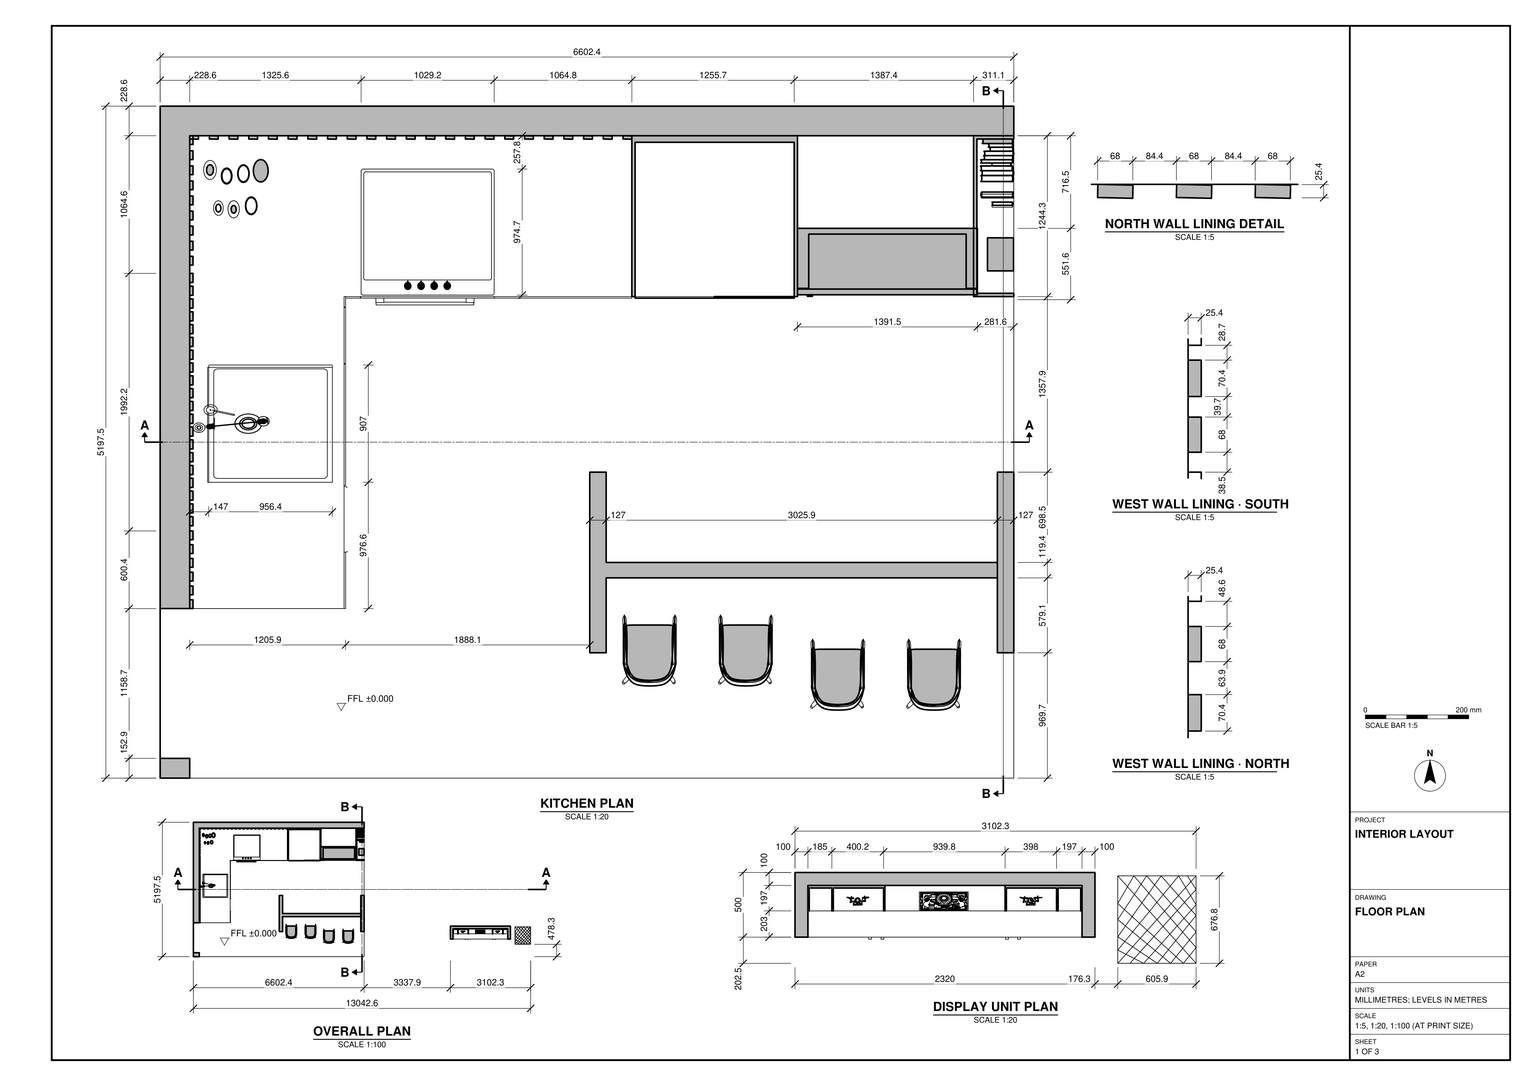
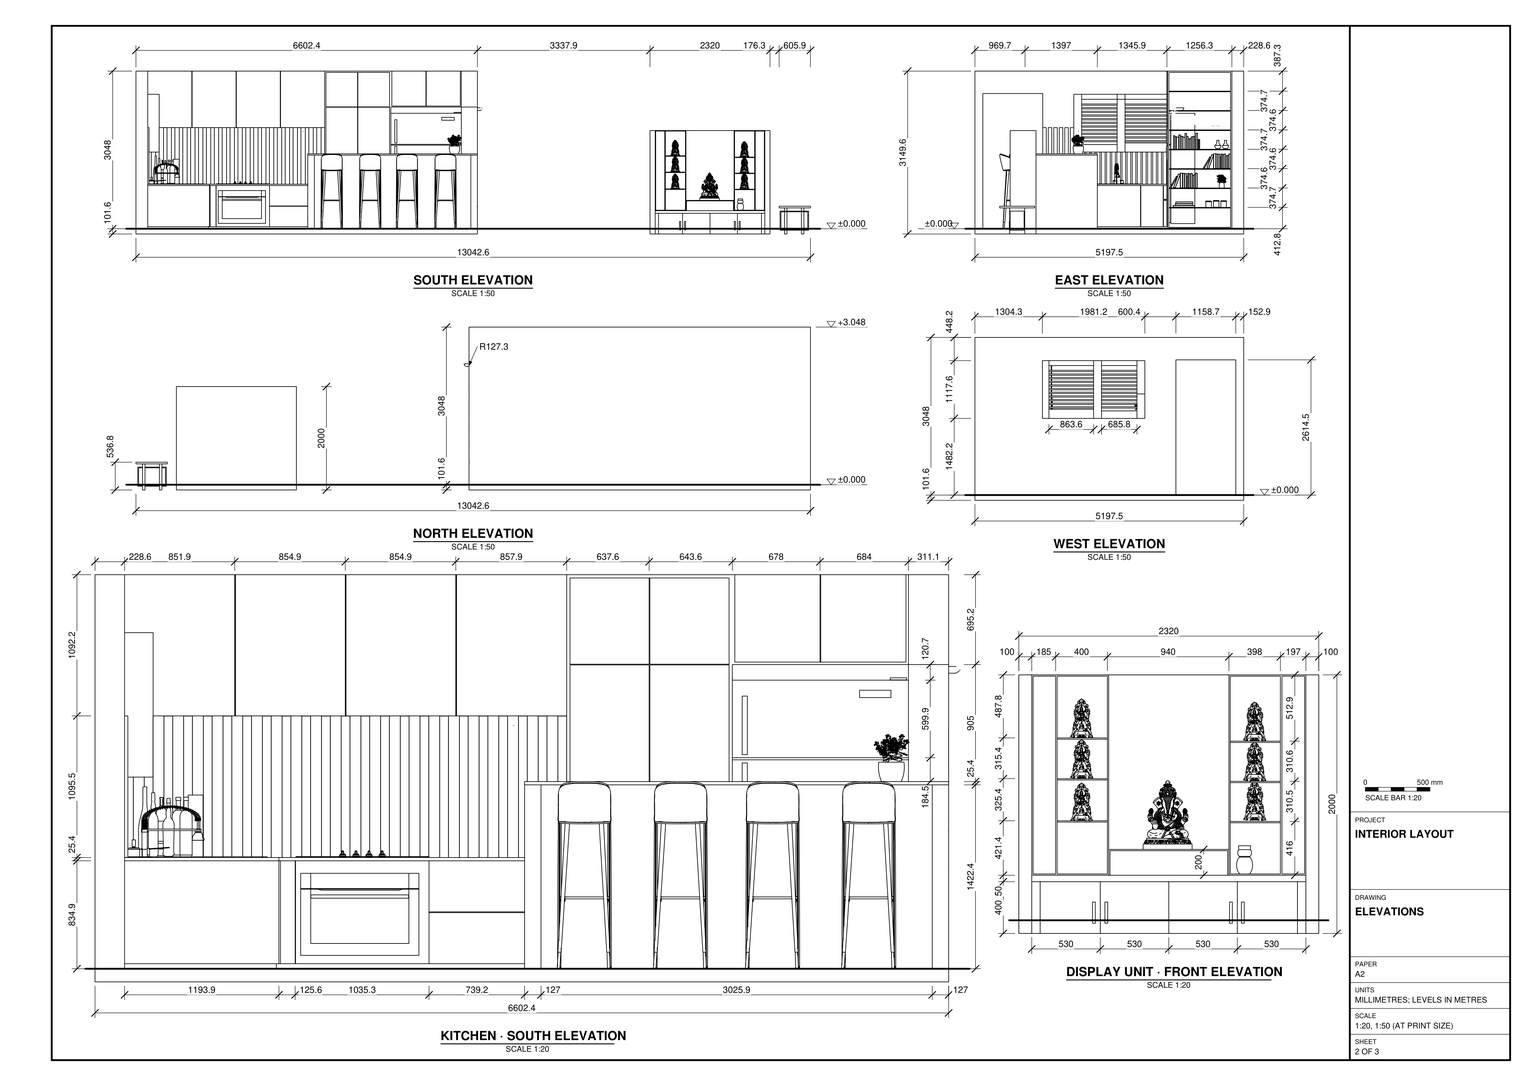
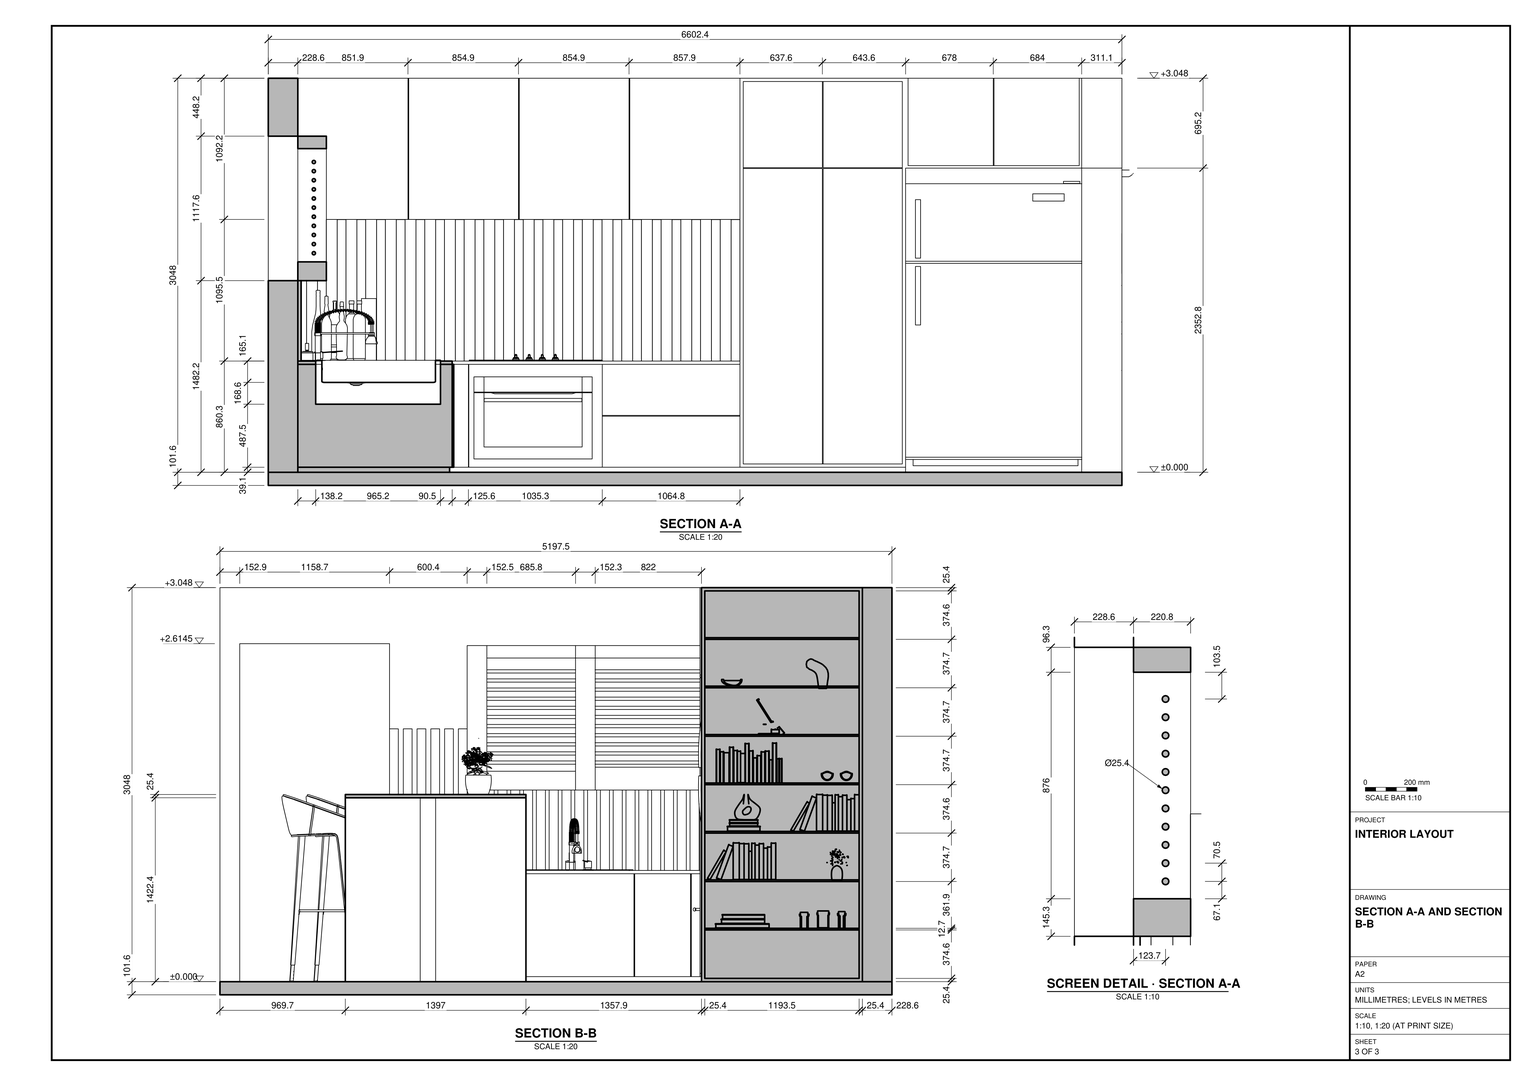
Build the interior in SketchUp from task_files/diagram_01.pdf. Work in millimetres and use the finished kitchen floor at ±0.000 (0 mm) as the level reference. The complete layout, including the display unit and the small table beyond it, measures 13042.6 mm along X, 5197.5 mm along Y and 3149.6 mm along Z.

Model the kitchen floor slab and the north and west walls with the thicknesses and openings shown. Use the plan details for the vertical wall lining and the west elevation and sections for the screened window. Form the L-shaped worktop with the sink and tap on the west return. Place the cooktop and oven along the north run, and match the base cabinet fronts, overhead cupboards, tall storage, refrigerator bay and end shelving to the elevations. In front of this run, model the raised bar with its end supports and four stools on the south side.

Use the overall plan to position the separate display unit and small table relative to the kitchen. Build the display unit with lower cupboards, narrow shelf bays on either side and a raised central display surface. Decor and loose items, including appliances, books, plants and display objects, may be any suitable library components placed as shown.

Keep walls, the slab and each furniture or joinery piece in separate groups or components, and use components for repeated parts. Save one SketchUp model as output_files/kitchen_interior_and_separate_display_unit.skp.

# SketchUp Ruby script. Lengths in millimetres.
U = 1.mm
M = Sketchup.active_model
def pt(a) = Geom::Point3d.new(a.map { |v| v * U })
def face(e, loops, mat)
  f = e.add_face(loops[0].map { |a| pt(a) })
  loops[1..].each { |l| e.add_face(l.map { |a| pt(a) }).erase! }
  f.material = f.back_material = mat if mat
  f
end
# faces: each face lists its corners as indices into pts; further lists are holes
def faces(e, pts, list, mat = nil) = list.each { |f| face(e, (f[0].is_a?(Array) ? f : [f]).map { |l| l.map { |i| pts[i] } }, mat) }
# xy, xz, yz: faces in a plane at the given z, y or x. An outline is a flat list of corners, or four numbers for a rectangle; further outlines are holes
def ring(l) = l.size == 4 ? [[l[0], l[1]], [l[2], l[1]], [l[2], l[3]], [l[0], l[3]]] : l.each_slice(2).to_a
def flat(e, list, mat, &to3) = list.each { |f| face(e, (f[0].is_a?(Array) ? f : [f]).map { |l| ring(l).map { |u, v| to3.(u, v) } }, mat) }
def xy(e, z, list, mat = nil) = flat(e, list, mat) { |x, y| [x, y, z] }
def xz(e, y, list, mat = nil) = flat(e, list, mat) { |x, z| [x, y, z] }
def yz(e, x, list, mat = nil) = flat(e, list, mat) { |y, z| [x, y, z] }
def lines(e, pts, list) = list.each { |a, b| e.add_line(pt(pts[a]), pt(pts[b])) }
# prism: a flat outline (further loops are holes) pulled along v
def prism(e, loops, v, mat = nil)
  f = face(e, loops, mat); d = Geom::Vector3d.new(v.map { |x| x * U })
  f.pushpull(f.normal.samedirection?(d) ? d.length : -d.length)
end
def box(e, o, s, mat = nil) = prism(e, [[o, [o[0] + s[0], o[1], o[2]], [o[0] + s[0], o[1] + s[1], o[2]], [o[0], o[1] + s[1], o[2]]]], [0, 0, s[2]], mat)
def at(x, y, z, deg = 0) = Geom::Transformation.translation(pt([x, y, z])) * Geom::Transformation.rotation(ORIGIN, Z_AXIS, deg.degrees)
def axes(o, x, y, z) = Geom::Transformation.new([*x, 0, *y, 0, *z, 0, *pt(o).to_a, 1])
def part(name) = M.definitions.add(name)
# library, detail: a bought-in or finely detailed component or shape, given as its bounding box
def library(name, o, s) = part(name).tap { |d| box(d.entities, o, s) }
def detail(e, o, s) = box(e.add_group.entities, o, s)
def put(e, d, t, mat = nil) = e.add_instance(d, t).tap { |i| i.material = mat if mat }
def group(e, t, mat = nil) = e.add_group.tap { |g| g.transformation = t; g.material = mat if mat }.entities
root = M.entities
M.materials.add("OAK TO USE 2").color = [202, 171, 128]
M.materials.add("PI964N").color = [18, 20, 26]
M.materials.add("VASO").color = [96, 96, 96]
M.materials.add("[Color C04]").color = [255, 153, 50]
M.materials.add("[Color D02]").color = [255, 229, 153]
M.materials.add("[Color M09]1").color = [0, 0, 0]
M.materials.add("[Wood Plywood Knots]").color = [137, 122, 41]
M.materials.add("stengel").color = [107, 129, 83]
M.materials.add("terracota").color = [125, 74, 68]
c1 = library("Component\#1",[0,0,0],[25.2,25.2,1727.2])
c2 = part("Component\#2")
box(c2.entities,[0,0,0],[25.4,68,1094.3])
c3 = library("Lavavajillas Drean Pro-Active",[-6.1,0.9,0],[598,573,820])
c4 = library("Bradanit 51U Blanc - Bradano - Evier sous plan - 54882",[0,0,-195],[550,420,200])
c5 = library("Pull-down kitchen faucet",[-39.4,-121.2,0],[342,375.6,427.3])
c6 = library("Untitled",[0,0,0],[595,626,595])
c7 = library("Beverage bottle collection",[0,0,0],[446.4,267.6,316])
c8 = library("PI964N",[0,0,-2],[600,513,30.4])
c9 = library("Oval planter",[0,0,0],[541.8,422.9,190])
c10 = library("Hanging philodendron",[-180.7,-260.1,-256],[931.9,931.9,1204.4])
c11 = library("Group145\#1",[149.2,164.2,242.8],[528.4,257.1,288.5])
c12 = library("Stack of books",[0,0,0],[415.7,278.4,106])
c13 = library("Architecture and design books\#1",[245.6,-0.5,0],[508.5,281.9,311.1])
c14 = library("book_4_k725760",[-2817.4,-1899.4,-325.7],[5634.8,3799,651.4])
c15 = library("Agrupar\#36",[-148.8,-110.2,0],[724.3,649.5,555.7])
c16 = library("Ganesha+-+An+Do+Giao",[214.1,-280.3,-3.5],[241.1,146.8,312])
c17 = library("GOD STATUE_1",[-396.2,-161.9,0],[792.4,323.8,999.5])
c18 = part("Difference")
xy(c18.entities,0,[[0,0,228.6,152.9],[0,1311.6,0,5197.5,6602.4,5197.5,6602.4,4968.9,228.6,4968.9,228.6,1311.6]])
xy(c18.entities,1482.2,[[0,1912,228.6,3893.2]])
xy(c18.entities,2599.8,[[0,1912,228.6,3893.2]])
xy(c18.entities,2614.5,[[0,152.9,228.6,1311.6]])
xy(c18.entities,3048,[[0,0,228.6,0,228.6,4968.9,6602.4,4968.9,6602.4,5197.5,0,5197.5]])
xz(c18.entities,0,[[0,0,228.6,3048]])
xz(c18.entities,152.9,[[0,0,228.6,2614.5]])
xz(c18.entities,1311.6,[[0,0,228.6,2614.5]])
xz(c18.entities,1912,[[0,1482.2,228.6,2599.8]])
xz(c18.entities,3893.2,[[0,1482.2,228.6,2599.8]])
xz(c18.entities,4968.9,[[228.6,0,6602.4,3048]])
xz(c18.entities,5197.5,[[0,0,6602.4,3048]])
yz(c18.entities,0,[[[0,0,0,3048,5197.5,3048,5197.5,0,1311.6,0,1311.6,2614.5,152.9,2614.5,152.9,0],[1912,1482.2,3893.2,2599.8]]])
yz(c18.entities,228.6,[[[0,0,152.9,0,152.9,2614.5,1311.6,2614.5,1311.6,0,4968.9,0,4968.9,3048,0,3048],[1912,1482.2,3893.2,2599.8]]])
yz(c18.entities,6602.4,[[4968.9,0,5197.5,3048]])
c19 = library("Group260",[-784.1,-474.7,-480.9],[1644.8,901.2,961.8])
c20 = library("Group\#31",[-33.1,-37.9,0],[338.4,315,385.4])
c21 = library("Group9",[-2292.8,-1935.4,0],[4572.5,3857.4,7040.1])
c22 = library("Group10",[-2671.6,-773.3,-1882.1],[5482.2,2177.2,4963.4])
c23 = library("Group11",[-3044.5,-1076.2,-3284.6],[6760.6,3266.6,7492.5])
c24 = library("Group21",[-3247.4,-2586,-500.4],[6494.8,5172.1,1000.8])
c25 = library("Group33",[-803.3,-828.6,-189.6],[2604.4,1657.2,1542.8])
c26 = library("Group\#663",[0,0,0],[241.8,541.5,348.6])
c27 = library("Group\#1447",[0,0,0],[115,115,159.9])
c28 = library("Group\#170",[0,0,0],[115,115,108.7])
c29 = library("Group\#1446",[0,0,0],[115,115,159.9])
c30 = library("Group\#175",[0,0,0],[272.5,119.3,108.7])
c31 = library("Group\#42",[0,0,0],[634,609.6,1728.8])
c32 = library("Group\#44",[0,0,0],[2320,500,2000])
c33 = library("Group\#45",[0,0,0],[2120,400,1600])
c34 = library("Group\#53",[0,0,0],[1584,1434,1773])
c35 = library("Group\#79",[0,0,0],[124,131.6,218.1])
box(root,[10509.9,664.8,78.9],[22,16,164])
box(root,[10605.9,664.8,78.9],[22,16,164])
box(root,[11569.9,664.8,78.9],[22,16,164])
box(root,[11661.9,664.8,78.9],[22,16,164])
xy(root,0,[[10040.3,680.8,12160.3,1080.8]])
xy(root,450,[[10635.3,883.8,11565.3,1080.8]])
xy(root,650,[[10635.3,883.8,11565.3,1080.8]],"[Color C04]")
xy(root,961.9,[[228.6,1951.7,254,2022.1],[228.6,2050.8,254,2121.2],[228.6,2149.8,254,2220.2],[228.6,2248.9,254,2319.3],[228.6,2348,254,2418.3],
  [228.6,2447,254,2517.4],[228.6,2546.1,254,2616.5],[228.6,2645.1,254,2715.5],[228.6,2744.2,254,2814.6],[228.6,2843.3,254,2913.6],
  [228.6,2942.3,254,3012.7],[228.6,3041.4,254,3111.8],[228.6,3140.4,254,3210.8],[228.6,3239.5,254,3309.9],[228.6,3338.6,254,3408.9],
  [228.6,3437.6,254,3508],[228.6,3536.7,254,3607.1],[228.6,3635.7,254,3706.1],[228.6,3734.8,254,3805.2],[228.6,3833.9,254,3904.2]])
xy(root,1583.8,[[228.6,1912,228.6,1951.7,254,1951.7,254,2022.1,228.6,2022.1,228.6,2050.8,254,2050.8,254,2064.4,449.4,2064.4,449.4,1912],[228.6,1951.7,254,2022.1],[228.6,2050.8,254,2064.4],[228.6,2064.4,254,2121.2],[254,2064.4,254,2121.2,228.6,2121.2,228.6,2149.8,254,2149.8,254,2220.2,228.6,2220.2,228.6,2248.9,254,2248.9,254,2319.3,228.6,2319.3,228.6,2348,254,2348,254,2418.3,228.6,2418.3,228.6,2447,254,2447,254,2517.4,228.6,2517.4,228.6,2546.1,254,2546.1,254,2616.5,228.6,2616.5,228.6,2645.1,254,2645.1,254,2715.5,228.6,2715.5,228.6,2744.2,254,2744.2,254,2750.2,449.4,2750.2,449.4,2064.4],
  [228.6,2149.8,254,2220.2],[228.6,2248.9,254,2319.3],[228.6,2348,254,2418.3],[228.6,2447,254,2517.4],[228.6,2546.1,254,2616.5],
  [228.6,2645.1,254,2715.5],[228.6,2744.2,254,2750.2],[228.6,2750.2,254,2814.6],[254,2750.2,254,2814.6,228.6,2814.6,228.6,2843.3,254,2843.3,254,2902.6,449.4,2902.6,449.4,2750.2],[228.6,2843.3,254,2902.6],
  [228.6,2902.6,254,2913.6],[254,2902.6,254,2913.6,228.6,2913.6,228.6,2942.3,254,2942.3,254,3012.7,228.6,3012.7,228.6,3041.4,254,3041.4,254,3111.8,228.6,3111.8,228.6,3140.4,254,3140.4,254,3210.8,228.6,3210.8,228.6,3239.5,254,3239.5,254,3309.9,228.6,3309.9,228.6,3338.6,254,3338.6,254,3408.9,228.6,3408.9,228.6,3437.6,254,3437.6,254,3508,228.6,3508,228.6,3536.7,254,3536.7,254,3607.1,228.6,3607.1,228.6,3635.7,254,3635.7,254,3706.1,228.6,3706.1,228.6,3734.8,254,3734.8,254,3766.2,449.4,3766.2,449.4,2902.6],[228.6,2942.3,254,3012.7],[228.6,3041.4,254,3111.8],[228.6,3140.4,254,3210.8],
  [228.6,3239.5,254,3309.9],[228.6,3338.6,254,3408.9],[228.6,3437.6,254,3508],[228.6,3536.7,254,3607.1],[228.6,3635.7,254,3706.1],
  [228.6,3734.8,254,3766.2],[228.6,3766.2,254,3805.2],[254,3766.2,254,3805.2,228.6,3805.2,228.6,3833.9,254,3833.9,254,3893.2,449.4,3893.2,449.4,3766.2],[228.6,3833.9,254,3893.2],[228.6,3893.2,254,3904.2]])
xy(root,1729.1,[[228.6,2064.4,449.4,2750.2]])
xy(root,1760.6,[[228.6,2902.6,449.4,3766.2]])
xy(root,2057.4,[[228.6,4182.2,1080.5,4194.2],[1086.5,4182.2,1935.4,4194.2],[1941.4,4182.2,2790.3,4194.2],[2796.3,4182.2,3648.2,4194.2],[228.6,4194.2,3648.2,4968.9]])
xy(root,2605.1,[[228.6,2064.4,449.4,2750.2],[228.6,2902.6,449.4,3766.2]])
xy(root,2701.4,[[228.6,1912,449.4,2064.4],[228.6,2064.4,449.4,2750.2],[228.6,2750.2,449.4,2902.6],[228.6,2902.6,449.4,3766.2],[228.6,3766.2,449.4,3893.2]])
xy(root,3149.6,[[228.6,4182.2,1080.5,4194.2],[1086.5,4182.2,1935.4,4194.2],[1941.4,4182.2,2790.3,4194.2],[2796.3,4182.2,3648.2,4194.2]])
xy(root,3149.6,[[228.6,4194.2,3648.2,4968.9]],"OAK TO USE 2")
xz(root,883.8,[[10645.3,450,11555.3,640]],"[Color C04]")
xz(root,883.8,[[10635.3,450,10645.3,450,10645.3,640,11555.3,640,11555.3,450,11565.3,450,11565.3,650,10635.3,650]],"[Color M09]1")
xz(root,1080.8,[[10635.3,450,11565.3,650]])
xz(root,1912,[[228.6,1583.8,449.4,2701.4]])
xz(root,1951.7,[[228.6,961.9,254,1583.8]],"[Wood Plywood Knots]")
xz(root,2022.1,[[228.6,961.9,254,1583.8]])
xz(root,2050.8,[[228.6,961.9,254,1583.8]],"[Wood Plywood Knots]")
xz(root,2064.4,[[228.6,1583.8,449.4,1729.1],[228.6,1729.1,449.4,2605.1],[228.6,2605.1,449.4,2701.4]])
xz(root,2121.2,[[228.6,961.9,254,1583.8]])
xz(root,2149.8,[[228.6,961.9,254,1583.8]],"[Wood Plywood Knots]")
xz(root,2220.2,[[228.6,961.9,254,1583.8]])
xz(root,2248.9,[[228.6,961.9,254,1583.8]],"[Wood Plywood Knots]")
xz(root,2319.3,[[228.6,961.9,254,1583.8]])
xz(root,2348,[[228.6,961.9,254,1583.8]],"[Wood Plywood Knots]")
xz(root,2418.3,[[228.6,961.9,254,1583.8]])
xz(root,2447,[[228.6,961.9,254,1583.8]])
xz(root,2517.4,[[228.6,961.9,254,1583.8]])
xz(root,2546.1,[[228.6,961.9,254,1583.8]])
xz(root,2616.5,[[228.6,961.9,254,1583.8]])
xz(root,2645.1,[[228.6,961.9,254,1583.8]])
xz(root,2715.5,[[228.6,961.9,254,1583.8]])
xz(root,2744.2,[[228.6,961.9,254,1583.8]])
xz(root,2750.2,[[228.6,1729.1,449.4,2605.1],[228.6,2605.1,449.4,2701.4]])
xz(root,2814.6,[[228.6,961.9,254,1583.8]])
xz(root,2843.3,[[228.6,961.9,254,1583.8]])
xz(root,2902.6,[[228.6,1583.8,449.4,1760.6],[228.6,1760.6,449.4,2605.1],[228.6,2605.1,449.4,2701.4]])
xz(root,2913.6,[[228.6,961.9,254,1583.8]])
xz(root,2942.3,[[228.6,961.9,254,1583.8]])
xz(root,3012.7,[[228.6,961.9,254,1583.8]])
xz(root,3041.4,[[228.6,961.9,254,1583.8]])
xz(root,3111.8,[[228.6,961.9,254,1583.8]])
xz(root,3140.4,[[228.6,961.9,254,1583.8]])
xz(root,3210.8,[[228.6,961.9,254,1583.8]])
xz(root,3239.5,[[228.6,961.9,254,1583.8]])
xz(root,3309.9,[[228.6,961.9,254,1583.8]])
xz(root,3338.6,[[228.6,961.9,254,1583.8]])
xz(root,3408.9,[[228.6,961.9,254,1583.8]])
xz(root,3437.6,[[228.6,961.9,254,1583.8]])
xz(root,3508,[[228.6,961.9,254,1583.8]])
xz(root,3536.7,[[228.6,961.9,254,1583.8]])
xz(root,3607.1,[[228.6,961.9,254,1583.8]])
xz(root,3635.7,[[228.6,961.9,254,1583.8]])
xz(root,3706.1,[[228.6,961.9,254,1583.8]])
xz(root,3734.8,[[228.6,961.9,254,1583.8]])
xz(root,3766.2,[[228.6,1760.6,449.4,2605.1],[228.6,2605.1,449.4,2701.4]])
xz(root,3805.2,[[228.6,961.9,254,1583.8]])
xz(root,3833.9,[[228.6,961.9,254,1583.8]])
xz(root,3893.2,[[228.6,1583.8,449.4,2701.4]])
xz(root,3904.2,[[228.6,961.9,254,1583.8]])
xz(root,4182.2,[[228.6,2057.4,1080.5,3149.6],[1086.5,2057.4,1935.4,3149.6],[1941.4,2057.4,2790.3,3149.6],[2796.3,2057.4,3648.2,3149.6]],"OAK TO USE 2")
xz(root,4194.2,[[228.6,2057.4,1080.5,3149.6],[1080.5,2057.4,1083.5,3149.6],[1083.5,2057.4,1086.5,3149.6],[1086.5,2057.4,1935.4,3149.6],[1935.4,2057.4,1938.4,3149.6],
  [1938.4,2057.4,1941.4,3149.6],[1941.4,2057.4,2790.3,3149.6],[2790.3,2057.4,2793.3,3149.6],[2793.3,2057.4,2796.3,3149.6],[2796.3,2057.4,3648.2,3149.6]])
xz(root,4968.9,[[228.6,2057.4,3648.2,3149.6]])
yz(root,0,[[152.9,101.6,1311.6,2716.1]])
yz(root,228.6,[[1951.7,961.9,2022.1,1583.8],[2050.8,961.9,2121.2,1583.8],[2149.8,961.9,2220.2,1583.8],[2248.9,961.9,2319.3,1583.8],[2348,961.9,2418.3,1583.8],
  [2447,961.9,2517.4,1583.8],[2546.1,961.9,2616.5,1583.8],[2645.1,961.9,2715.5,1583.8],[2744.2,961.9,2814.6,1583.8],[2843.3,961.9,2913.6,1583.8],
  [2942.3,961.9,3012.7,1583.8],[3041.4,961.9,3111.8,1583.8],[3140.4,961.9,3210.8,1583.8],[3239.5,961.9,3309.9,1583.8],[3338.6,961.9,3408.9,1583.8],
  [3437.6,961.9,3508,1583.8],[3536.7,961.9,3607.1,1583.8],[3635.7,961.9,3706.1,1583.8],[3734.8,961.9,3805.2,1583.8],[3833.9,961.9,3904.2,1583.8],
  [1912,1583.8,2064.4,2057.4],[2064.4,1583.8,2750.2,1729.1],[2750.2,1583.8,2902.6,2701.4],[2902.6,1583.8,3766.2,1760.6],[3766.2,1583.8,3893.2,2701.4],
  [1912,2057.4,2064.4,2701.4],[4182.2,2057.4,4194.2,3149.6],[4194.2,2057.4,4968.9,3149.6],[2064.4,2605.1,2750.2,2701.4],[2902.6,2605.1,3766.2,2701.4]])
yz(root,254,[[1951.7,961.9,2022.1,1583.8],[2050.8,961.9,2121.2,1583.8],[2149.8,961.9,2220.2,1583.8],[2248.9,961.9,2319.3,1583.8],[2348,961.9,2418.3,1583.8],
  [2447,961.9,2517.4,1583.8],[2546.1,961.9,2616.5,1583.8],[2645.1,961.9,2715.5,1583.8],[2744.2,961.9,2814.6,1583.8],[2843.3,961.9,2913.6,1583.8],
  [2942.3,961.9,3012.7,1583.8],[3041.4,961.9,3111.8,1583.8],[3140.4,961.9,3210.8,1583.8],[3239.5,961.9,3309.9,1583.8],[3338.6,961.9,3408.9,1583.8],
  [3437.6,961.9,3508,1583.8],[3536.7,961.9,3607.1,1583.8],[3635.7,961.9,3706.1,1583.8],[3734.8,961.9,3805.2,1583.8],[3833.9,961.9,3904.2,1583.8]],"[Wood Plywood Knots]")
yz(root,449.4,[[1912,1583.8,2064.4,2701.4],[2064.4,1583.8,2750.2,1729.1],[2750.2,1583.8,2902.6,2605.1],[2902.6,1583.8,3766.2,1760.6],[3766.2,1583.8,3893.2,2701.4],
  [2064.4,2605.1,2750.2,2701.4],[2750.2,2605.1,2902.6,2701.4],[2902.6,2605.1,3766.2,2701.4]])
yz(root,1080.5,[[4182.2,2057.4,4194.2,3149.6]])
yz(root,1086.5,[[4182.2,2057.4,4194.2,3149.6]])
yz(root,1935.4,[[4182.2,2057.4,4194.2,3149.6]])
yz(root,1941.4,[[4182.2,2057.4,4194.2,3149.6]])
yz(root,2790.3,[[4182.2,2057.4,4194.2,3149.6]])
yz(root,2796.3,[[4182.2,2057.4,4194.2,3149.6]])
yz(root,3648.2,[[4182.2,2057.4,4194.2,3149.6],[4194.2,2057.4,4968.9,3149.6]])
yz(root,10635.3,[[883.8,450,1080.8,650]])
yz(root,11565.3,[[883.8,450,1080.8,650]])
p = [[3236.3,2002.1,1982.3],[3236.3,2002,1982.4],[3236.2,2002.1,1982.4],[3236.2,2002.1,1982.3],[3236.4,2001,1983.8],[3236.6,2000.4,1984.8],
  [3236.5,2001.3,1983.7],[228.6,4182.2,2057.4],[228.6,3893.2,2057.4],[228.6,3932.9,961.9],[228.6,4003.3,961.9]]
faces(root,p,[[0,1,2,3],[6,1,5],[1,4,6],[6,4,5]],"stengel")
faces(root,p,[[1,4,5]])
lines(root,p,[[7,8],[9,10]])
put(root,c1,axes([364.9,2064.4,2489],[-1,0,0],[0,0,1],[0,1,0]))
put(root,c1,axes([364.9,2064.4,2418.5],[-1,0,0],[0,0,1],[0,1,0]))
put(root,c1,axes([364.9,2064.4,2348],[-1,0,0],[0,0,1],[0,1,0]))
put(root,c1,axes([364.9,2064.4,2277.4],[-1,0,0],[0,0,1],[0,1,0]))
put(root,c1,axes([364.9,2064.4,2206.9],[-1,0,0],[0,0,1],[0,1,0]))
put(root,c1,axes([364.9,2064.4,2136.3],[-1,0,0],[0,0,1],[0,1,0]))
put(root,c1,axes([364.9,2064.4,2065.8],[-1,0,0],[0,0,1],[0,1,0]))
put(root,c1,axes([364.9,2064.4,1995.2],[-1,0,0],[0,0,1],[0,1,0]))
put(root,c1,axes([364.9,2064.4,1924.7],[-1,0,0],[0,0,1],[0,1,0]))
put(root,c1,axes([364.9,2064.4,1854.2],[-1,0,0],[0,0,1],[0,1,0]))
put(root,c1,axes([364.9,2064.4,1783.6],[-1,0,0],[0,0,1],[0,1,0]))
put(root,c2,at(228.6,1311.6,963.1),"[Wood Plywood Knots]")
put(root,c2,at(228.6,1418.1,963.1),"[Wood Plywood Knots]")
put(root,c2,at(228.6,1524.5,963.1),"[Wood Plywood Knots]")
put(root,c2,at(228.6,1631,963.1),"[Wood Plywood Knots]")
put(root,c2,at(228.6,1737.5,963.1),"[Wood Plywood Knots]")
put(root,c2,at(228.6,1844,963.1),"[Wood Plywood Knots]")
put(root,c2,at(228.6,3968.1,961.9))
put(root,c2,at(228.6,4084.7,961.9),"[Wood Plywood Knots]")
put(root,c2,at(228.6,4201.3,961.9),"[Wood Plywood Knots]")
put(root,c2,at(228.6,4317.9,961.9),"[Wood Plywood Knots]")
put(root,c2,at(228.6,4434.5,961.9),"[Wood Plywood Knots]")
put(root,c2,at(228.6,4551.1,961.9),"[Wood Plywood Knots]")
put(root,c2,at(228.6,4667.7,961.9),"[Wood Plywood Knots]")
put(root,c2,at(228.6,4784.3,961.9),"[Wood Plywood Knots]")
put(root,c2,at(228.6,4900.9,961.9))
put(root,c2,at(228.6,4968.9,961.9,-91.3))
put(root,c2,at(380.9,4968.9,961.9,-91.3),"[Wood Plywood Knots]")
put(root,c2,at(533.3,4968.9,961.9,-91.3),"[Wood Plywood Knots]")
put(root,c2,at(685.6,4968.9,961.9,-91.3),"[Wood Plywood Knots]")
put(root,c2,at(838,4968.9,961.9,-91.3),"[Wood Plywood Knots]")
put(root,c2,at(990.3,4968.9,961.9,-91.3),"[Wood Plywood Knots]")
put(root,c2,at(1142.7,4968.9,961.9,-91.3),"[Wood Plywood Knots]")
put(root,c2,at(1295,4968.9,961.9,-91.3),"[Wood Plywood Knots]")
put(root,c2,at(1447.4,4968.9,961.9,-91.3),"[Wood Plywood Knots]")
put(root,c2,at(1599.7,4968.9,961.9,-91.3),"[Wood Plywood Knots]")
put(root,c2,at(1752.1,4968.9,961.9,-91.3),"[Wood Plywood Knots]")
put(root,c2,at(1904.4,4968.9,961.9,-91.3),"[Wood Plywood Knots]")
put(root,c2,at(2056.8,4968.9,961.9,-91.3),"[Wood Plywood Knots]")
put(root,c2,at(2209.1,4968.9,961.9,-91.3),"[Wood Plywood Knots]")
put(root,c2,at(2361.5,4968.9,961.9,-91.3),"[Wood Plywood Knots]")
put(root,c2,at(2513.8,4968.9,961.9,-91.3),"[Wood Plywood Knots]")
put(root,c2,at(2666.1,4968.9,961.9,-91.3),"[Wood Plywood Knots]")
put(root,c2,at(2818.5,4968.9,961.9,-91.3),"[Wood Plywood Knots]")
put(root,c2,at(2970.8,4968.9,961.9,-91.3),"[Wood Plywood Knots]")
put(root,c2,at(3123.2,4968.9,961.9,-91.3),"[Wood Plywood Knots]")
put(root,c2,at(3275.5,4968.9,961.9,-91.3),"[Wood Plywood Knots]")
put(root,c2,at(3427.9,4968.9,961.9,-91.3),"[Wood Plywood Knots]")
put(root,c2,at(3580.2,4968.9,961.9,-91.3),"[Wood Plywood Knots]")
put(root,c3,axes([1446.5,1752.2,140.7],[0,0.85,0],[-1.04,0,0],[0,0,0.97054]))
put(root,c4,axes([375.7,3195.2,963],[0,-1.64915,0],[2.27691,0,0],[0,0,0.97837]))
put(root,c5,axes([243.9,2684.4,958.4],[1.98656,-0.4157,0],[0.51746,1.59589,0],[0,0,0.94835]))
put(root,c6,axes([1590.8,3659.9,204.8],[1.53681,0,0],[0,0.90735,0],[0,0,1.06723]))
put(root,c7,axes([336.3,4784.7,961.9],[1.118,0,0],[0,-1.68912,0],[0,0,1.73146]))
put(root,c8,axes([1554.2,3736.3,964],[1.71533,0,0],[0,1.9,0],[0,0,2]))
put(root,c9,axes([6602.4,3793,2387.6],[-0.31027,0.31027,0],[0.28962,0.28962,0],[0,0,0.27305]),"terracota")
put(root,c10,axes([6531.6,3810.4,2249.6],[0.57077,-0.05716,0],[0.07517,0.57285,0],[0,0,0.3777]))
put(root,c11,at(6766.6,4265.9,1020.8,90))
put(root,c11,at(6766.6,3621.2,646.2,90))
put(root,c12,at(6602.4,3831.6,514.3,90))
put(root,c13,at(6601.9,3592.7,1638.3,90))
put(root,c14,axes([6522.1,4050.6,1315.4],[0,0.03937,0],[-0.03937,0,0],[0,0,0.03937]))
put(root,c14,axes([6522.1,4050.6,1341.2],[0,0.03937,0],[-0.03937,0,0],[0,0,0.03937]))
put(root,c15,axes([6384.4,4660,880.9],[0.49248,0,0],[0,0.49248,0],[0,0,0.49248]),"VASO")
put(root,c16,axes([10565.7,1164.1,656.1],[1.57,0,0],[0,1,0],[0,0,1.71]))
put(root,c17,axes([10427,963.6,861.4],[0.21682,0,0],[0,0.2303,0],[0,0,0.30361]))
put(root,c17,axes([10427,963.6,1196.8],[0.21682,0,0],[0,0.2303,0],[0,0,0.30361]))
put(root,c17,axes([10427,963.6,1512.2],[0.21682,0,0],[0,0.2303,0],[0,0,0.30361]))
put(root,c17,axes([11765,963.6,1487.6],[0.21682,0,0],[0,0.2303,0],[0,0,0.30361]))
put(root,c17,axes([11765,963.6,1178.1],[0.21682,0,0],[0,0.2303,0],[0,0,0.30361]))
put(root,c17,axes([11765,963.6,872.6],[0.21682,0,0],[0,0.2303,0],[0,0,0.30361]))
g1 = group(root,at(0,0,0))
box(g1,[0,0,0],[6602.4,5197.5,101.6])
put(root,c18,at(0,0,101.6))
g2 = group(root,at(228.6,1379.5,101.6),"OAK TO USE 2")
xy(g2,0,[[0,-68,0,3589.3,4700.7,3589.3,4700.7,2365,1173.9,2365,1173.9,-68],[6062.7,2345,6373.8,3589.3]])
xy(g2,25.4,[[6088.1,2370.4,6373.8,3563.9]])
xy(g2,39.1,[[0,-68,1173.9,0],[1173.9,-68,1193.9,0],[1193.9,-68,1205.9,367.6],[0,0,1173.9,0,1173.9,2365,1193.9,2365,1193.9,3589.3,0,3589.3],[1173.9,0,1193.9,2345],
  [1193.9,885.4,1205.9,1822.5],[1193.9,1828.5,1205.9,2260.2],[1193.9,2266.2,1205.9,2345],[2354.8,2333,3419.6,2333,3419.6,2345,4700.7,2345,4700.7,2365,1193.9,2365,1193.9,2345,2354.8,2345],[1205.9,2333,1319.5,2345],
  [1322.5,2333,2354.8,2345],[1173.9,2345,1193.9,2365],[1193.9,2365,4700.7,3589.3]])
xy(g2,64.5,[[3445,2333,4057.1,2345],[4063.1,2333,4675.3,2345],[3445,2345,4675.3,3538.5]])
xy(g2,103.2,[[1362.2,2333,2276.6,2345],[1362.2,2345,2276.6,3538.5]])
xy(g2,400,[[6088.1,2370.4,6373.8,3563.9]])
xy(g2,412.7,[[6088.1,2370.4,6373.8,3563.9]])
xy(g2,434,[[2354.8,2333,3419.6,2345]])
xy(g2,440,[[2354.8,2333,3419.6,2345]])
xy(g2,526.6,[[138.2,908.7,1103.4,1797.7]])
xy(g2,738.2,[[1362.2,2333,2276.6,2345],[1362.2,2345,2276.6,3538.5]])
xy(g2,774.7,[[6088.1,2370.4,6373.8,3563.9]])
xy(g2,787.4,[[6088.1,2370.4,6373.8,3563.9]])
xy(g2,834.9,[[0,-68,1193.9,0],[1193.9,-68,1205.9,367.6],[[0,0,1193.9,3589.3],[138.2,908.7,1103.4,1797.7]],[1193.9,885.4,1205.9,1822.5],[1193.9,1828.5,1205.9,2260.2],
  [1193.9,2266.2,1205.9,2345],[1205.9,2333,1319.5,2345],[1322.5,2333,2354.8,2345],[2354.8,2333,3419.6,2345],[1193.9,2345,3419.6,3589.3]])
xy(g2,860.3,[[[0,-68,1193.9,-68,1193.9,2345,3419.6,2345,3419.6,3589.3,0,3589.3],[138.2,908.7,1103.4,1797.7]]])
xy(g2,1149.3,[[6088.1,2370.4,6373.8,3563.9]])
xy(g2,1162,[[6088.1,2370.4,6373.8,3563.9]])
xy(g2,1524,[[6088.1,2370.4,6373.8,3563.9]])
xy(g2,1536.7,[[6088.1,2370.4,6373.8,3563.9]])
xy(g2,1898.6,[[6088.1,2370.4,6373.8,3563.9]])
xy(g2,1911.3,[[6088.1,2370.4,6373.8,3563.9]])
xy(g2,2273.3,[[6088.1,2370.4,6373.8,3563.9]])
xy(g2,2286,[[6088.1,2370.4,6373.8,3563.9]])
xy(g2,2349.8,[[3445,2333,4057.1,2345],[4063.1,2333,4675.3,2345]])
xy(g2,2352.8,[[4700.7,2345,6062.7,3589.3]])
xy(g2,2355.8,[[3445,2333,4057.1,2345],[4063.1,2333,4675.3,2345]])
xy(g2,2372,[[4719.8,2333,5378.7,2345],[4719.8,2345,6043.5,3538.5]])
xy(g2,2647.9,[[6088.1,2370.4,6373.8,3563.9]])
xy(g2,2660.6,[[6088.1,2370.4,6373.8,3563.9]])
xy(g2,3022.6,[[3445,2333,4057.1,2345],[4063.1,2333,4675.3,2345],[3445,2345,4675.3,3538.5],[6088.1,2370.4,6373.8,3563.9]])
xy(g2,3048,[[4719.8,2333,5378.7,2345],[3419.6,2345,4700.7,3589.3],[4700.7,2345,4719.8,2345,4719.8,3538.5,6043.5,3538.5,6043.5,2345,6062.7,2345,6062.7,3589.3,4700.7,3589.3],[4719.8,2345,6043.5,3538.5],[6062.7,2345,6373.8,3589.3]])
xz(g2,-68,[[0,0,1173.9,39.1],[0,39.1,1193.9,834.9],[1193.9,39.1,1205.9,834.9],[0,834.9,1193.9,860.3]])
xz(g2,0,[[0,39.1,1193.9,834.9]])
xz(g2,367.6,[[1193.9,39.1,1205.9,834.9]])
xz(g2,885.4,[[1193.9,39.1,1205.9,834.9]])
xz(g2,908.7,[[138.2,526.6,1103.4,834.9],[138.2,834.9,1103.4,860.3]])
xz(g2,1797.7,[[138.2,526.6,1103.4,834.9],[138.2,834.9,1103.4,860.3]])
xz(g2,1822.5,[[1193.9,39.1,1205.9,834.9]])
xz(g2,1828.5,[[1193.9,39.1,1205.9,834.9]])
xz(g2,2260.2,[[1193.9,39.1,1205.9,834.9]])
xz(g2,2266.2,[[1193.9,39.1,1205.9,834.9]])
xz(g2,2333,[[1205.9,39.1,1319.5,834.9],[[1322.5,39.1,2354.8,834.9],[1362.2,103.2,2276.6,738.2]],[2354.8,39.1,3419.6,434],[2354.8,440,3419.6,834.9],[4719.8,2372,5378.7,3048]])
xz(g2,2333,[[3445,64.5,4057.1,2349.8],[4063.1,64.5,4675.3,2349.8],[3445,2355.8,4057.1,3022.6],[4063.1,2355.8,4675.3,3022.6]],"OAK TO USE 2")
xz(g2,2345,[[6062.7,0,6373.8,2352.8],[1193.9,39.1,1205.9,834.9],[1205.9,39.1,1319.5,834.9],[1319.5,39.1,1322.5,834.9],[[1322.5,39.1,2354.8,834.9],[1362.2,103.2,2276.6,738.2]],
  [[3419.6,39.1,4700.7,39.1,4700.7,2352.8,6062.7,2352.8,6062.7,3048,6043.5,3048,6043.5,2372,4719.8,2372,4719.8,3048,3419.6,3048],[3445,64.5,4675.3,3022.6]],[4057.1,64.5,4063.1,64.5,4063.1,2349.8,4675.3,2349.8,4675.3,2355.8,4063.1,2355.8,4063.1,3022.6,4057.1,3022.6,4057.1,2355.8,3445,2355.8,3445,2349.8,4057.1,2349.8],[4063.1,64.5,4675.3,2349.8],[2354.8,434,3419.6,440],[1193.9,834.9,3419.6,860.3],
  [6062.7,2352.8,6373.8,3048],[3445,2355.8,4057.1,3022.6],[4063.1,2355.8,4675.3,3022.6],[4719.8,2372,5378.7,3048],[5378.7,2372,5384.7,3048],
  [5384.7,2372,6043.5,3048]])
xz(g2,2365,[[1173.9,0,4700.7,39.1]])
xz(g2,2370.4,[[6088.1,25.4,6373.8,412.7],[6088.1,412.7,6373.8,787.4],[6088.1,787.4,6373.8,1162],[6088.1,1162,6373.8,1536.7],[6088.1,1536.7,6373.8,1911.3],
  [6088.1,1911.3,6373.8,2286],[6088.1,2286,6373.8,2660.6],[6088.1,2660.6,6373.8,3022.6]])
xz(g2,3538.5,[[3445,64.5,4675.3,3022.6],[1362.2,103.2,2276.6,738.2],[4719.8,2372,6043.5,3048]])
xz(g2,3563.9,[[6088.1,25.4,6373.8,412.7],[6088.1,412.7,6373.8,787.4],[6088.1,787.4,6373.8,1162],[6088.1,1162,6373.8,1536.7],[6088.1,1536.7,6373.8,1911.3],
  [6088.1,1911.3,6373.8,2286],[6088.1,2286,6373.8,2660.6],[6088.1,2660.6,6373.8,3022.6]])
xz(g2,3589.3,[[0,0,4700.7,39.1],[6062.7,0,6373.8,2352.8],[1193.9,39.1,1193.9,834.9,3419.6,834.9,3419.6,3048,4700.7,3048,4700.7,39.1],[0,834.9,3419.6,860.3],[4700.7,2352.8,6373.8,3048]])
yz(g2,0,[[-68,0,3589.3,39.1],[-68,39.1,0,834.9],[-68,834.9,3589.3,860.3]])
yz(g2,138.2,[[908.7,526.6,1797.7,834.9],[908.7,834.9,1797.7,860.3]])
yz(g2,1103.4,[[908.7,526.6,1797.7,834.9],[908.7,834.9,1797.7,860.3]])
yz(g2,1173.9,[[-68,0,2365,39.1]])
yz(g2,1193.9,[[-68,39.1,0,834.9],[0,39.1,367.6,834.9],[367.6,39.1,370.6,834.9],[370.6,39.1,373.6,834.9],[879.4,39.1,882.4,834.9],
  [882.4,39.1,885.4,834.9],[885.4,39.1,1822.5,834.9],[1822.5,39.1,1825.5,834.9],[1825.5,39.1,1828.5,834.9],[1825.5,39.1,1828.5,834.9],
  [1828.5,39.1,2260.2,834.9],[2260.2,39.1,2263.2,834.9],[2263.2,39.1,2266.2,834.9],[2266.2,39.1,2345,834.9],[-68,834.9,2345,860.3]])
yz(g2,1205.9,[[-68,39.1,367.6,834.9],[885.4,39.1,1822.5,834.9],[1828.5,39.1,2260.2,834.9],[2266.2,39.1,2333,834.9],[2333,39.1,2345,834.9]])
yz(g2,1319.5,[[2333,39.1,2345,834.9]])
yz(g2,1322.5,[[2333,39.1,2345,834.9]])
yz(g2,1362.2,[[2333,103.2,2345,738.2],[2345,103.2,3538.5,738.2]])
yz(g2,2276.6,[[2333,103.2,2345,738.2],[2345,103.2,3538.5,738.2]])
yz(g2,2354.8,[[2333,39.1,2345,434],[2333,434,2345,440],[2333,440,2345,834.9]])
yz(g2,3419.6,[[2333,39.1,2345,434],[2333,440,2345,834.9],[2345,834.9,3589.3,860.3],[2345,860.3,3589.3,3048]])
yz(g2,3445,[[2333,64.5,2345,834.9],[2345,64.5,3538.5,834.9],[2333,834.9,2345,860.3],[2345,834.9,3538.5,860.3],[2333,860.3,2345,2349.8],
  [2345,860.3,3538.5,3022.6],[2333,2355.8,2345,3022.6]])
yz(g2,4057.1,[[2333,64.5,2345,2349.8],[2333,2355.8,2345,3022.6]])
yz(g2,4063.1,[[2333,64.5,2345,2349.8],[2333,2355.8,2345,3022.6]])
yz(g2,4675.3,[[2333,64.5,2345,2349.8],[2345,64.5,3538.5,2352.8],[2345,2352.8,3538.5,3022.6],[2333,2355.8,2345,3022.6]])
yz(g2,4700.7,[[2365,0,3589.3,39.1],[2345,39.1,3589.3,2352.8]])
yz(g2,4719.8,[[2333,2372,2345,3048],[2345,2372,3538.5,3048]])
yz(g2,5378.7,[[2333,2372,2345,3048]])
yz(g2,6043.5,[[2345,2372,3538.5,3048]])
yz(g2,6062.7,[[2345,0,3589.3,2352.8]])
yz(g2,6088.1,[[2370.4,25.4,3563.9,412.7],[2370.4,412.7,3563.9,787.4],[2370.4,787.4,3563.9,1162],[2370.4,1162,3563.9,1536.7],[2370.4,1536.7,3563.9,1911.3],
  [2370.4,1911.3,3563.9,2286],[2370.4,2286,3563.9,2660.6],[2370.4,2660.6,3563.9,3022.6]])
yz(g2,6373.8,[[[2345,0,3589.3,3048],[2370.4,25.4,3563.9,3022.6]],[2370.4,400,3563.9,412.7],[2370.4,774.7,3563.9,787.4],[2370.4,1149.3,3563.9,1162],[2370.4,1524,3563.9,1536.7],
  [2370.4,1898.6,3563.9,1911.3],[2370.4,2273.3,3563.9,2286],[2370.4,2647.9,3563.9,2660.6]])
g3 = group(root,at(6475.4,969.7,101.6))
box(g3,[0,0,0],[127,1397,1422.4])
g4 = group(root,at(3322.6,969.7,101.6))
prism(g4,[[[0,1397,0],[127,1397,0],[127,698.5,0],[3152.9,698.5,0],[3152.9,579.1,0],[127,579.1,0],[127,0,0],[0,0,0]]],[0,0,1422.4])
g5 = group(root,at(3322.6,969.7,1524))
box(g5,[0,0,0],[3279.9,1397,25.4])
put(root,c19,axes([4119.5,993.9,825.5],[1,0,0],[0,1.23,0],[0,0,1.50528]))
put(root,c19,axes([5575.3,806.9,825.5],[1,0,0],[0,1.23,0],[0,0,1.50528]))
put(root,c20,at(6025.9,1870.5,1549.4))
put(root,c21,axes([6504.5,4236.9,2014.2],[0,0.03937,0],[-0.03937,0,0],[0,0,0.03937]))
put(root,c22,axes([6522.2,4067.9,1428.1],[0,0.03937,0],[-0.03937,0,0],[0,0,0.03937]))
put(root,c23,axes([6574.8,4559.2,2499.5],[0,0.03937,0],[-0.03937,0,0],[0,0,0.03937]))
put(root,c24,axes([6500.6,4051.2,1283.3],[0,0.03937,0],[-0.03937,0,0],[0,0,0.03937]))
put(root,c25,axes([6522.7,4295,2021],[0,0.03937,0],[-0.03937,0,0],[0,0,0.03937]))
put(root,c26,axes([6423.7,4637.2,1638.3],[0.49357,0,0],[0,0.49357,0],[0,0,0.49357]))
put(root,c27,axes([6532,4866.6,509.4],[-1,0,0],[0,-1,0],[0,0,0.84072]))
put(root,c28,axes([6535.3,4576.3,510.2],[-1,0,0],[0,-1,0],[0,0,1.17429]))
put(root,c29,axes([6548,4722.9,514.3],[-1,0,0],[0,-1,0],[0,0,0.84072]))
put(root,c30,axes([6423.4,4751.9,2013],[0,-0.71,0],[0.71,0,0],[0,0,0.71]))
put(root,c31,axes([4929.3,4252.4,152.4],[0,-0.87,0],[2.28266,0,0],[0,0,1.2723]))
put(root,c32,at(9940.3,680.8,0))
put(root,c33,at(10040.3,680.8,400),"[Color D02]")
put(root,c34,axes([12436.7,478.3,0],[0.38254,0,0],[0,0.47196,0],[0,0,0.30278]))
put(root,c35,at(11624.5,916.8,460))
